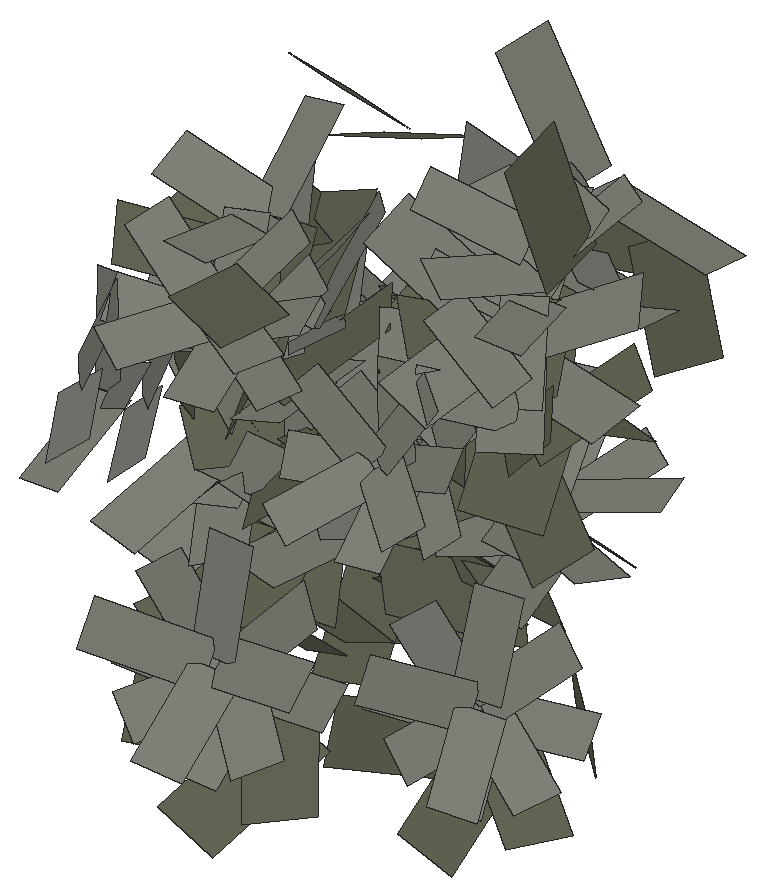
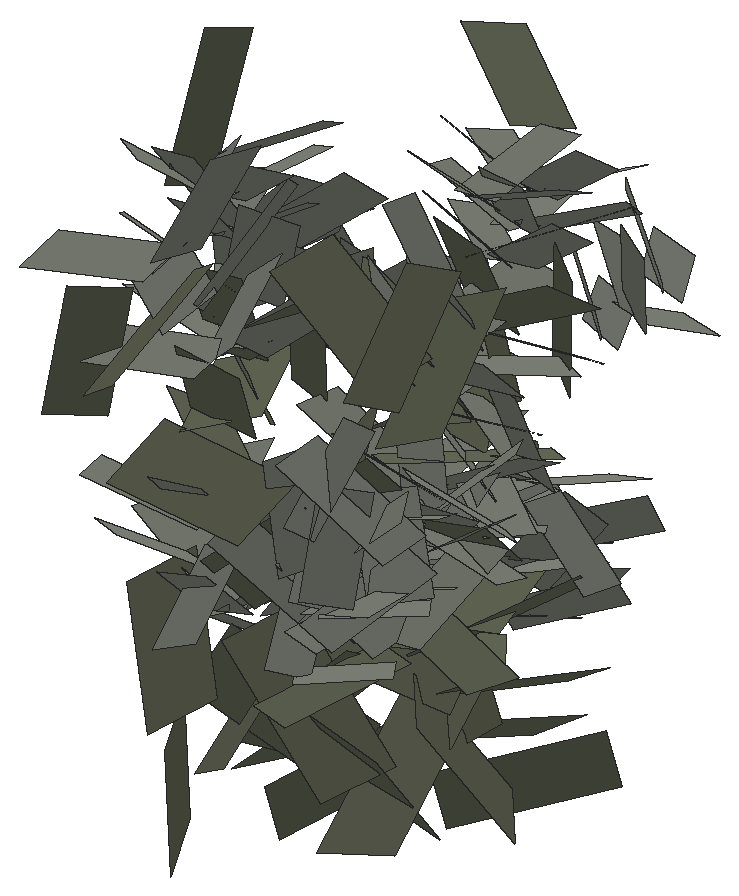
# SketchUp Ruby script. Lengths in inches.
U = 1.inch
M = Sketchup.active_model
def pt(a) = Geom::Point3d.new(a.map { |v| v * U })
def face(e, loops, mat)
  f = e.add_face(loops[0].map { |a| pt(a) })
  loops[1..].each { |l| e.add_face(l.map { |a| pt(a) }).erase! }
  f.material = f.back_material = mat if mat
  f
end
# faces: each face lists its corners as indices into pts; further lists are holes
def faces(e, pts, list, mat = nil) = list.each { |f| face(e, (f[0].is_a?(Array) ? f : [f]).map { |l| l.map { |i| pts[i] } }, mat) }
# xy, xz, yz: faces in a plane at the given z, y or x. An outline is a flat list of corners, or four numbers for a rectangle; further outlines are holes
def ring(l) = l.size == 4 ? [[l[0], l[1]], [l[2], l[1]], [l[2], l[3]], [l[0], l[3]]] : l.each_slice(2).to_a
def flat(e, list, mat, &to3) = list.each { |f| face(e, (f[0].is_a?(Array) ? f : [f]).map { |l| ring(l).map { |u, v| to3.(u, v) } }, mat) }
def xy(e, z, list, mat = nil) = flat(e, list, mat) { |x, y| [x, y, z] }
def xz(e, y, list, mat = nil) = flat(e, list, mat) { |x, z| [x, y, z] }
def yz(e, x, list, mat = nil) = flat(e, list, mat) { |y, z| [x, y, z] }
def lines(e, pts, list) = list.each { |a, b| e.add_line(pt(pts[a]), pt(pts[b])) }
# prism: a flat outline (further loops are holes) pulled along v
def prism(e, loops, v, mat = nil)
  f = face(e, loops, mat); d = Geom::Vector3d.new(v.map { |x| x * U })
  f.pushpull(f.normal.samedirection?(d) ? d.length : -d.length)
end
def box(e, o, s, mat = nil) = prism(e, [[o, [o[0] + s[0], o[1], o[2]], [o[0] + s[0], o[1] + s[1], o[2]], [o[0], o[1] + s[1], o[2]]]], [0, 0, s[2]], mat)
def at(x, y, z, deg = 0) = Geom::Transformation.translation(pt([x, y, z])) * Geom::Transformation.rotation(ORIGIN, Z_AXIS, deg.degrees)
def axes(o, x, y, z) = Geom::Transformation.new([*x, 0, *y, 0, *z, 0, *pt(o).to_a, 1])
def part(name) = M.definitions.add(name)
# library, detail: a bought-in or finely detailed component or shape, given as its bounding box
def library(name, o, s) = part(name).tap { |d| box(d.entities, o, s) }
def detail(e, o, s) = box(e.add_group.entities, o, s)
def put(e, d, t, mat = nil) = e.add_instance(d, t).tap { |i| i.material = mat if mat }
def group(e, t, mat = nil) = e.add_group.tap { |g| g.transformation = t; g.material = mat if mat }.entities
root = M.entities
M.materials.add("viburnumblaasdfas0df1w06d").color = [98, 102, 84]
M.materials.add("viburnumbladsadfasdfad0w122").color = [125, 129, 119]
c1 = part("Component\#315")
p = [[0.25,0,0],[2.05,0.01,0.35],[1.81,4.2,1.66],[0,4.19,1.3125]]
faces(c1.entities,p,[[0,1,2,3]],"viburnumbladsadfasdfad0w122")
c2 = part("viburnumblad2")
put(c2.entities,c1,axes([-19.23,-4.49,-32.18],[83.35428,0,0],[0,79.38502,0],[0,0,83.35428]))
c3 = part("Component\#314")
p = [[0.14,0,0],[2.58,0.05,0.25],[2.44,5.11,2.64],[0,5.05,2.39]]
faces(c3.entities,p,[[0,1,2,3]],"viburnumblaasdfas0df1w06d")
c4 = part("viburnumblad1\#2")
put(c4.entities,c3,axes([-37.25,6.23,19.31],[75.98784,0,0],[0,65.50676,0],[0,0,75.98784]))
put(root,c2,axes([1226.33,274.85,14.94],[0.00016,-0.01206,-0.00411],[0.01207,-0.0013,0.00429],[-0.00443,-0.00391,0.01129]))
put(root,c2,axes([1229.25,283.21,16.14],[-0.01389,0,-0.00185],[-0.00005,-0.01523,0.00032],[-0.00201,0.00032,0.0151]))
put(root,c4,axes([1228.82,284.94,25.53],[-0.01366,0.00026,0.00163],[0.00037,-0.01516,0.00432],[0.00177,0.00434,0.01188]))
put(root,c2,axes([1227.91,269.2,22.33],[0.01118,-0.00278,0.00257],[-0.00082,0.00655,0.0102],[-0.00357,-0.00931,0.00467]))
put(root,c2,axes([1226.33,278.8,18.92],[0.00883,-0.00666,-0.00546],[0.00861,0.00836,0.00373],[0.00207,-0.0066,0.01002]))
put(root,c2,axes([1229.81,277.7,17.24],[0.00207,0.01081,-0.00198],[-0.01024,0.00263,0.00364],[0.00398,0.00114,0.01039]))
put(root,c4,axes([1230.33,279.36,10.75],[-0.01218,0.00376,0.00725],[-0.00872,-0.0119,-0.00846],[0.0032,-0.00977,0.01045]))
put(root,c4,axes([1230.91,277.52,4.82],[-0.00011,0.00616,0.01357],[-0.0165,-0.00475,0.00202],[0.00445,-0.01294,0.00591]))
put(root,c4,axes([1227.07,278.17,5.83],[0.01021,-0.01095,0.0021],[0.01009,0.01114,0.00903],[-0.00698,-0.00405,0.01279]))
put(root,c4,axes([1225.9,281.68,13.5],[-0.00229,-0.01326,-0.00295],[0.0155,-0.0021,-0.00237],[0.00206,-0.00324,0.01267]))
put(root,c2,axes([1230,275.96,15.39],[-0.0137,0.00216,0.00156],[-0.00229,-0.00943,-0.00711],[-0.00005,-0.00804,0.01068]))
put(root,c2,axes([1226.58,279.63,17.48],[0.00038,-0.01114,-0.00561],[0.01301,0.00109,-0.00087],[0.0016,-0.0057,0.01058]))
put(root,c2,axes([1230.72,284.14,17.18],[-0.00604,0.00926,-0.00001],[-0.00892,-0.00582,-0.00295],[-0.00247,-0.0016,0.01066]))
put(root,c2,axes([1231.21,274.45,23.76],[-0.00263,0.0123,0.00535],[-0.01296,-0.00091,-0.00426],[-0.00348,-0.00589,0.01184]))
put(root,c2,axes([1229.125,277.97,15.94],[0.00864,0.00566,-0.00294],[-0.00615,0.01026,0.00169],[0.00342,0.0003,0.01064]))
put(root,c2,axes([1230.12,273.79,17.89],[-0.01312,0.00207,0.00149],[-0.00255,-0.01047,-0.0079],[-0.00005,-0.00804,0.01068]))
put(root,c2,axes([1227.85,278.78,18.53],[-0.00829,-0.0091,-0.00248],[0.00914,-0.00728,-0.00415],[0.002,-0.00468,0.01099]))
put(root,c2,axes([1230.34,285.84,17.18],[-0.01091,0.00229,-0.00461],[-0.00339,-0.01305,0.00154],[-0.00434,0.00249,0.01152]))
put(root,c2,axes([1229.875,268.62,22.7],[-0.01118,0.00278,-0.00257],[-0.00011,-0.00839,-0.00838],[-0.00365,-0.00753,0.00688]))
put(root,c2,axes([1230.76,277.88,18.45],[-0.00607,0.00939,0.00026],[-0.0086,-0.00567,0.00435],[0.00378,0.00216,0.0103]))
put(root,c2,axes([1230.97,283.08,17.18],[0.00229,0.01091,-0.00461],[-0.01305,0.00339,0.00154],[0.00249,0.00434,0.01152]))
put(root,c2,axes([1227.89,274.44,18.43],[0.01312,-0.00207,-0.00149],[0.00246,0.00822,0.01025],[-0.00067,-0.01033,0.00845]))
put(root,c4,axes([1229.13,282.68,22.59],[-0.01489,-0.00148,0.00524],[0.00198,-0.01828,0.00047],[0.00517,0.00094,0.01496]))
put(root,c2,axes([1227.68,268.5625,23.79],[0.00814,-0.00715,-0.0046],[0.00716,0.00216,0.00888],[-0.00455,-0.00881,0.00477]))
put(root,c2,axes([1229.48,278.42,18.7],[0.009,0.00589,-0.00306],[-0.00569,0.0095,0.00156],[0.00342,0.0003,0.01064]))
put(root,c4,axes([1231.67,274.02,22.86],[0.0051,0.011,0.00655],[-0.01483,0.00551,0.0023],[-0.00067,-0.00681,0.01196]))
put(root,c4,axes([1232.05,277.62,10.8],[-0.00702,0.01204,0.00725],[-0.01547,-0.00958,0.00093],[0.00442,-0.0058,0.01392]))
put(root,c2,axes([1228.73,284.16,17.9],[-0.01077,-0.01069,-0.00135],[0.00977,-0.00996,0.00094],[-0.00168,-0.00022,0.01514]))
put(root,c4,axes([1229.32,272.61,20.55],[0.01089,-0.00679,0.00142],[0.00218,0.00667,0.0129],[-0.00665,-0.00902,0.00468]))
put(root,c2,axes([1231.39,284.74,14.59],[-0.0063,0.00967,-0.00001],[-0.00803,-0.00524,-0.00265],[-0.00247,-0.0016,0.01066]))
put(root,c2,axes([1229.08,268.06,23.91],[-0.00766,-0.00322,-0.00823],[0.00764,-0.00813,-0.00386],[-0.0046,-0.00755,0.00633]))
put(root,c2,axes([1231.57,276.66,14.33],[0.00051,0.01437,0.00412],[-0.01266,-0.00025,0.00242],[0.00266,-0.00396,0.0135]))
put(root,c2,axes([1231.73,283.59,18.58],[-0.007,0.00987,-0.00339],[-0.01018,-0.00558,0.00479],[0.00226,0.00542,0.01111]))
put(root,c4,axes([1229.17,280.28,6.07],[0.01682,-0.00022,0.00237],[-0.00091,0.01794,0.00812],[-0.00224,-0.00704,0.0153]))
put(root,c2,axes([1231.18,275.52,22.14],[0.00694,0.00883,0.00779],[-0.01027,0.00714,0.00105],[-0.0037,-0.00696,0.01117]))
put(root,c2,axes([1232.01,275.5,17.65],[0.00048,0.01376,0.00394],[-0.01406,-0.00028,0.00269],[0.00266,-0.00396,0.0135]))
put(root,c2,axes([1229.83,286.6,18.58],[-0.00987,-0.007,-0.00339],[0.00558,-0.01018,0.00479],[-0.00542,0.00226,0.01111]))
put(root,c2,axes([1231.8,272.82,28.14],[0.00044,0.0126,0.00361],[-0.0113,0.00031,0.00032],[0.00024,-0.00347,0.01207]))
put(root,c2,axes([1232.23,276.08,20.97],[-0.00274,0.01284,0.00559],[-0.01166,-0.00082,-0.00384],[-0.00348,-0.00589,0.01184]))
put(root,c4,axes([1230.46,284.3,6.45],[-0.01776,-0.00139,0.00308],[0.00179,-0.02087,0.00087],[0.003,0.001,0.0178]))
put(root,c4,axes([1228.36,278.68,13.14],[0.01107,-0.00525,0.00049],[0.00612,0.01279,-0.0012],[0,0.00115,0.01221]))
put(root,c4,axes([1232.75,273.61,25.15],[-0.0066,0.01089,0.00527],[-0.0139,-0.00777,-0.00135],[0.00164,-0.00514,0.01268]))
put(root,c2,axes([1228.74,269.65,23.34],[0.00034,-0.00733,-0.00907],[0.00978,-0.00348,0.00299],[-0.00497,-0.00808,0.00546]))
put(root,c2,axes([1230.03,275.71,23.9],[0.01244,0.00019,0.00567],[-0.00322,0.01148,0.00668],[-0.00467,-0.00741,0.01049]))
put(root,c2,axes([1231.07,278.27,16.84],[-0.01065,0.00247,0.00234],[-0.00174,-0.01065,0.00331],[0.00294,0.00276,0.01043]))
put(root,c2,axes([1228.8,270.61,22.42],[0.0085,-0.00746,-0.0048],[0.00645,0.00195,0.00799],[-0.00455,-0.00881,0.00477]))
put(root,c2,axes([1232.09,271.56,10.17],[-0.00011,0.00779,0.00854],[-0.01208,-0.00262,0.00224],[0.00345,-0.0089,0.00816]))
put(root,c2,axes([1227.92,284.33,19.89],[0,-0.01516,-0.00154],[0.01507,-0.00022,0.00221],[-0.00223,-0.00152,0.015]))
put(root,c2,axes([1228.24,284.51,16.125],[0,-0.01583,-0.00161],[0.01357,-0.0002,0.00199],[-0.00223,-0.00152,0.015]))
put(root,c2,axes([1231.55,285.12,16.15],[-0.01032,0.0026,-0.00299],[-0.00231,-0.01123,-0.0018],[-0.0033,-0.001,0.0105]))
put(root,c2,axes([1229.9,275.68,17.3125],[-0.01106,-0.0052,-0.00541],[0.00776,-0.00965,-0.0066],[-0.00127,-0.0082,0.01048]))
put(root,c2,axes([1229.21,278.8125,17.22],[0.01065,-0.00247,-0.00234],[0.00251,0.01145,-0.00069],[0.00243,0.00013,0.01091]))
put(root,c2,axes([1232.61,275.64,22.875],[-0.01065,0.00857,-0.00023],[-0.00787,-0.00997,-0.00669],[-0.00415,-0.00484,0.01209]))
put(root,c4,axes([1233.78,278.32,15.75],[0.00121,0.01104,0.01007],[-0.01675,0.00403,-0.00241],[-0.00386,-0.00953,0.01091]))
put(root,c2,axes([1231.18,276.36,16.01],[0.01044,0.00958,0.00206],[-0.00879,0.00856,0.00474],[0.00211,-0.00514,0.0132]))
put(root,c2,axes([1232.86,276.46,15.95],[-0.00976,0.00988,0.00351],[-0.01076,-0.01049,-0.00039],[0.00219,-0.00277,0.01388]))
put(root,c2,axes([1229.97,270.15,22.62],[-0.00655,-0.0022,-0.00816],[0.00764,-0.00813,-0.00386],[-0.0054,-0.00785,0.00541]))
put(root,c4,axes([1230.25,278.77,13.42],[-0.01365,-0.00518,-0.0014],[0.0059,-0.01311,-0.00908],[0.00168,-0.00777,0.01232]))
put(root,c2,axes([1228.44,275.99,17.59],[0.00749,-0.00812,-0.00752],[0.01093,0.00403,0.00654],[-0.00171,-0.00982,0.0089]))
put(root,c2,axes([1232.49,269.22,12.02],[0.00026,0.00745,0.01011],[-0.01208,-0.00262,0.00224],[0.00344,-0.00977,0.00711]))
put(root,c2,axes([1231.48,270.58,11.4],[0.00896,0.00627,0.00619],[-0.00837,0.00305,0.00903],[0.00298,-0.01046,0.00629]))
put(root,c4,axes([1232.73,285.58,12.23],[-0.011,0.00511,-0.00003],[-0.00581,-0.01252,-0.00271],[-0.00101,-0.0021,0.0119]))
put(root,c2,axes([1232.85,269.78,25.04],[-0.00261,0.00974,0.006],[-0.01123,-0.00353,0.00072],[0.00254,-0.00551,0.00899]))
put(root,c2,axes([1232.17,270.71,24.1],[0.00601,0.00853,0.00433],[-0.01051,0.00446,0.00545],[0.00235,-0.00645,0.00846]))
put(root,c2,axes([1232.1,269.15,26.35],[0.00626,0.00889,0.00451],[-0.00973,0.00413,0.00504],[0.00235,-0.00645,0.00846]))
put(root,c4,axes([1229.4375,278.43,8.47],[-0.00936,-0.00715,0.0061],[0.00985,-0.01174,0.00135],[0.00403,0.00472,0.01172]))
put(root,c4,axes([1234.13,277.57,18.41],[-0.01024,0.01003,0.00441],[-0.01249,-0.0094,-0.00763],[-0.00202,-0.00765,0.01274]))
put(root,c4,axes([1228.52,283.75,25.59],[-0.00484,-0.01365,0.00231],[0.016,-0.00575,-0.00049],[0.00117,0.00203,0.01447]))
put(root,c2,axes([1230.64,278.92,15.56],[-0.00842,-0.00565,0.00174],[0.00635,-0.00914,0.00106],[0.00096,0.00194,0.01097]))
put(root,c4,axes([1231.02,276.02,20.64],[0.01421,-0.00084,0.00442],[-0.0012,0.01582,0.00687],[-0.00438,-0.00595,0.01294]))
put(root,c2,axes([1232.34,284.63,19.83],[-0.01229,0.00259,0.00001],[-0.00225,-0.0107,0.00618],[0.00128,0.00604,0.01094]))
put(root,c2,axes([1229.17,277.08,16.37],[-0.00242,-0.00904,-0.00878],[0.01402,-0.00344,-0.00033],[-0.00196,-0.00893,0.00974]))
put(root,c2,axes([1231.15,277.07,21.14],[0.01184,0.00091,0.00415],[-0.00322,0.01148,0.00668],[-0.0033,-0.00735,0.01104]))
put(root,c2,axes([1229.42,274.91,18.94],[-0.00252,-0.00942,-0.00914],[0.01298,-0.00318,-0.00031],[-0.00196,-0.00893,0.00974]))
put(root,c2,axes([1229.51,279.32,15.7],[0.00633,-0.0098,-0.00027],[0.00833,0.00542,-0.00155],[0.00159,0.00072,0.01104]))
put(root,c2,axes([1231.17,285.39,17.62],[-0.00856,-0.00558,-0.00422],[0.00556,-0.00947,0.00126],[-0.00425,-0.00115,0.01014]))
put(root,c4,axes([1228.69,279.24,10.95],[0.00308,-0.0114,0.00333],[0.01375,0.00318,-0.00182],[0.00071,0.00361,0.0117]))
put(root,c2,axes([1233.23,270.8,11.1875],[-0.00859,0.00427,0.00811],[-0.00794,-0.00683,-0.00482],[0.00302,-0.00917,0.00803]))
put(root,c4,axes([1232.6,276.16,6.97],[-0.01186,-0.00066,0.00699],[-0.00532,-0.01121,-0.01007],[0.00532,-0.0098,0.0081]))
put(root,c2,axes([1232.3,275.37,24.74],[-0.01244,-0.00019,-0.00567],[0.00199,-0.01294,-0.00394],[-0.00531,-0.00441,0.0118]))
put(root,c2,axes([1230.67,277.8125,14.84],[0.01298,0.00037,-0.00224],[0.00059,0.01317,0.00559],[0.0024,-0.0056,0.01296]))
put(root,c2,axes([1230.21,279.59,16.85],[-0.00207,-0.01081,0.00198],[0.01001,-0.00209,-0.00093],[0.00139,0.00174,0.01096]))
put(root,c2,axes([1231.24,279.17,18.16],[-0.009,-0.00589,0.00306],[0.00635,-0.00914,0.00106],[0.00195,0.00259,0.0107]))
put(root,c4,axes([1229.22,285.53,9.72],[-0.00613,-0.01546,0.00166],[0.01796,-0.00686,0.00247],[-0.00138,0.00232,0.01649]))
put(root,c2,axes([1230.99,273.87,28.45],[0.01156,-0.00022,-0.00012],[0.00026,0.01157,0.0049],[0.00003,-0.0049,0.01157]))
put(root,c2,axes([1229.96,279.71,18.4],[0.00607,-0.00939,-0.00026],[0.00926,0.00603,-0.00173],[0.00159,0.00072,0.01104]))
put(root,c2,axes([1231.74,286.05,14.97],[-0.00821,-0.00536,-0.00406],[0.00601,-0.01023,0.00136],[-0.00425,-0.00115,0.01014]))
put(root,c4,axes([1231.34,273.01,22.41],[0.01287,-0.00107,0.00071],[0.00034,0.01171,0.00907],[-0.00141,-0.0079,0.00892]))
put(root,c2,axes([1233.59,269.3,26.27],[-0.00995,0.00489,0.00397],[-0.00607,-0.00954,-0.00338],[0.0019,-0.00477,0.00949]))
put(root,c2,axes([1233,277.79,14.51],[-0.01371,0.0002,0.00098],[-0.0004,-0.01527,-0.00242],[0.00098,-0.00226,0.01411]))
put(root,c2,axes([1231.02,276.93,18.14],[0.01428,-0.00021,-0.00102],[0.00059,0.01317,0.00559],[0.00086,-0.00561,0.01315]))
put(root,c2,axes([1233.05,273.75,28.49],[-0.01199,0.00073,-0.00108],[-0.00063,-0.01339,-0.00213],[-0.00123,-0.0019,0.01236]))
put(root,c4,axes([1230.57,274.58,20.49],[0.00428,-0.01029,-0.00658],[0.01194,-0.00078,0.00879],[-0.00649,-0.00737,0.00685]))
put(root,c2,axes([1231.79,270.43,25.51],[0.01146,0.00283,0.00038],[-0.00257,0.0094,0.00741],[0.00146,-0.00704,0.00821]))
put(root,c2,axes([1230.79,277.23,22.93],[0.01065,-0.00857,0.00023],[0.00633,0.00812,0.0092],[-0.00584,-0.00699,0.01019]))
put(root,c2,axes([1233.15,272.25,10.67],[-0.01296,-0.00148,0.00142],[-0.00002,-0.00776,-0.00823],[0.00196,-0.00903,0.00851]))
put(root,c4,axes([1233.6,280.8,13.54],[0.01304,-0.00033,0.00964],[-0.00605,0.01553,0.00873],[-0.00811,-0.00915,0.01066]))
put(root,c2,axes([1233.52,276.48,17.84],[-0.01428,0.00021,0.00102],[-0.00037,-0.01414,-0.00224],[0.00098,-0.00226,0.01411]))
put(root,c2,axes([1231.62,269.89,13.17],[0.01241,0.00141,-0.00136],[0.00049,0.00618,0.01093],[0.0019,-0.01085,0.00605]))
put(root,c2,axes([1233.24,277.13,21.93],[-0.01194,-0.00018,-0.00545],[0.00215,-0.01397,-0.00426],[-0.00531,-0.00441,0.0118]))
put(root,c2,axes([1232.27,284.98,17.97],[-0.01038,-0.0062,0.0034],[0.00714,-0.00931,0.00482],[0.00014,0.00586,0.01111]))
put(root,c2,axes([1231.125,276.625,24.875],[0.00263,-0.0123,-0.00535],[0.01173,-0.00054,0.007],[-0.00651,-0.00594,0.01045]))
put(root,c2,axes([1233.79,269.91,12.62],[-0.01241,-0.00141,0.00136],[-0.00002,-0.00862,-0.00914],[0.00196,-0.00903,0.00851]))
put(root,c4,axes([1235.05,281.62,7.9375],[0.0025,0.01316,0.00583],[-0.01545,-0.00015,0.00696],[0.00546,-0.00635,0.01198]))
put(root,c2,axes([1231.41,284.98,16.52],[-0.00213,-0.01089,0.00325],[0.01232,-0.002,0.0014],[-0.00076,0.00372,0.01198]))
put(root,c4,axes([1235.48,282.8,14.21],[0.00442,0.01183,0.01203],[-0.01827,-0.00182,0.0085],[0.00605,-0.01272,0.01028]))
put(root,c2,axes([1232.42,277.02,23.55],[-0.00694,-0.00883,-0.00779],[0.00996,-0.00923,0.0016],[-0.00629,-0.00487,0.01112]))
put(root,c4,axes([1232.12,283.44,15.36],[-0.01205,-0.00086,0.01408],[0.00278,-0.02131,0.00108],[0.0139,0.00242,0.01204]))
put(root,c2,axes([1233.84,270.82,25.53],[-0.01146,-0.00283,-0.00038],[0.00275,-0.01049,-0.00491],[0.00082,-0.00467,0.00968]))
put(root,c2,axes([1231.97,271.95,24.9],[0.01038,-0.0051,-0.00415],[0.00572,0.00729,0.00502],[0.00038,-0.00694,0.0084]))
put(root,c2,axes([1231.25,278.29,16.61],[0.00976,-0.00988,-0.00351],[0.01058,0.00912,0.00376],[-0.00035,-0.00511,0.01338]))
put(root,c4,axes([1230.84,282.71,8.77],[-0.00166,-0.01224,0.00834],[0.01717,-0.00122,0.00163],[-0.00056,0.00844,0.01227]))
put(root,c4,axes([1232.74,275.85,19.44],[-0.00918,-0.00626,-0.00848],[0.01129,-0.01094,-0.00412],[-0.00395,-0.00772,0.00939]))
put(root,c2,axes([1232.03,270.43,27.11],[0.00995,-0.00489,-0.00397],[0.00635,0.0081,0.00558],[0.00038,-0.00694,0.0084]))
put(root,c2,axes([1231.75,271.54,12.66],[0.00859,-0.00427,-0.00811],[0.00913,0.005,0.00703],[0.00084,-0.0107,0.00653]))
put(root,c4,axes([1232.7,275.16,9.32],[-0.01126,-0.00753,-0.00255],[0.00827,-0.00884,-0.01044],[0.00351,-0.00867,0.01012]))
put(root,c4,axes([1231.57,275.07,21.39],[0.0077,-0.00971,-0.00377],[0.01191,0.00736,0.00523],[-0.00177,-0.00557,0.01033]))
put(root,c2,axes([1233.06,278,16.41],[-0.01044,-0.00958,-0.00206],[0.0098,-0.01029,-0.00181],[-0.00027,-0.00273,0.01406]))
put(root,c4,axes([1235.23,281.32,4.53],[-0.00036,0.00539,0.01277],[-0.01275,-0.00915,0.0035],[0.00843,-0.01005,0.00448]))
put(root,c2,axes([1233.14,271.65,12.4],[-0.00896,-0.00627,-0.00619],[0.0092,-0.00573,-0.00751],[0.00088,-0.00942,0.00827]))
put(root,c2,axes([1232.43,271.52,26.07],[0.00261,-0.00974,-0.006],[0.01057,0.00192,0.00135],[-0.00026,-0.0062,0.0089]))
put(root,c2,axes([1232.14,272.89,11.74],[-0.00025,-0.00716,-0.0097],[0.01356,0.0002,-0.00049],[0.00042,-0.01011,0.00745]))
put(root,c2,axes([1233.23,272.08,24.93],[-0.00572,-0.00761,-0.00506],[0.01001,-0.00557,-0.00285],[-0.00075,-0.00619,0.00889]))
put(root,c4,axes([1235.39,285.26,8.43],[-0.01278,0.00636,0.00656],[-0.00548,-0.01653,0.00535],[0.00782,0.00178,0.01351]))
put(root,c2,axes([1233.51,270.57,27.03],[-0.00626,-0.00889,-0.00451],[0.01001,-0.00557,-0.00285],[-0.00007,-0.00526,0.00943]))
put(root,c2,axes([1232.53,277.91,18.32],[-0.00048,-0.01376,-0.00394],[0.01429,-0.00069,0.00066],[-0.00082,-0.00391,0.01375]))
put(root,c2,axes([1232.92,270.58,13.76],[-0.00026,-0.00745,-0.01011],[0.01255,0.00018,-0.00046],[0.00042,-0.01011,0.00745]))
put(root,c4,axes([1232.83,276.46,19.46],[-0.00628,-0.01206,-0.00336],[0.01448,-0.00668,-0.00311],[0.00091,-0.00388,0.01211]))
put(root,c4,axes([1236.89,281.75,9.93],[-0.00888,0.00849,0.00791],[-0.01054,-0.01309,0.0022],[0.00721,-0.00377,0.01214]))
put(root,c2,axes([1237.17,280.76,13.2],[-0.00337,0.01279,0.00428],[-0.0107,-0.00403,0.00361],[0.00507,-0.00269,0.01202]))
put(root,c4,axes([1233.54,269.74,28.38],[-0.00662,-0.01127,-0.00498],[0.01432,-0.00702,-0.0031],[-0.00011,-0.00548,0.01154]))
put(root,c2,axes([1236.76,286.43,14.33],[-0.01437,0.00051,0.00412],[0.00025,-0.01266,0.00242],[0.00396,0.00266,0.0135]))
put(root,c2,axes([1237.11,280.38,14.79],[0.0065,0.01157,0.00112],[-0.00968,0.00489,0.00566],[0.0049,-0.00389,0.01176]))
put(root,c2,axes([1238.04,272.59,20.04],[-0.00143,0.00635,0.00868],[-0.0108,-0.00196,-0.00037],[0.00136,-0.00839,0.00553]))
put(root,c2,axes([1237.23,271.65,20.95],[0.00668,0.00514,0.00687],[-0.00864,0.00277,0.00603],[0.00109,-0.00897,0.00475]))
put(root,c2,axes([1238.28,279.87,16.18],[-0.00323,0.01225,0.0041],[-0.01189,-0.00447,0.00401],[0.00507,-0.00269,0.01202]))
put(root,c2,axes([1238.1,278.0625,21.99],[0.00298,0.01174,0.00601],[-0.01309,-0.0001,0.00669],[0.00586,-0.00729,0.01134]))
put(root,c2,axes([1237.56,273.82,19.61],[0.00642,0.00493,0.0066],[-0.00933,0.00299,0.00651],[0.00109,-0.00897,0.00475]))
put(root,c4,axes([1237.97,281.84,16.59],[-0.01126,0.00378,0.01091],[-0.00977,-0.0152,-0.00482],[0.00789,-0.0086,0.01113]))
put(root,c2,axes([1236.1,281.51,13.8125],[0.01096,0.00423,-0.00348],[-0.00277,0.01177,0.00559],[0.00527,-0.00421,0.01149]))
put(root,c2,axes([1238.16,282.06,25.57],[-0.00842,0.01125,0.00685],[-0.00786,-0.01092,0.00827],[0.01063,0.001,0.01143]))
put(root,c2,axes([1238.54,280.97,14.55],[-0.01106,0.00576,0.00468],[-0.00631,-0.01247,0.00042],[0.00435,-0.00178,0.01246]))
put(root,c4,axes([1233.21,284.99,18.66],[-0.00321,-0.01557,0.00645],[0.01613,-0.00714,-0.00921],[0.00952,0.00374,0.01377]))
put(root,c2,axes([1238.62,271.63,20.89],[-0.00871,0.00384,0.00541],[-0.00663,-0.00614,-0.00616],[0.00084,-0.00787,0.00624]))
put(root,c4,axes([1239.03,278.47,20.96],[0.00193,0.01121,0.0059],[-0.01433,0.00039,0.00396],[0.00283,-0.0062,0.01085]))
put(root,c2,axes([1238.38,281.88,27.91],[0.00042,0.01563,0.00009],[-0.01107,0.00024,0.01104],[0.01103,-0.00036,0.01108]))
put(root,c2,axes([1237.49,283.14,23.89],[-0.01223,0.0001,0.00757],[0.00075,-0.01555,0.00142],[0.00819,0.0016,0.01322]))
put(root,c2,axes([1238.66,276.43,9.12],[-0.00143,0.00682,0.00818],[-0.0095,-0.00594,0.0033],[0.00662,-0.0068,0.00682]))
put(root,c2,axes([1238.98,276.12,24.79],[0.00385,0.0119,0.00772],[-0.01309,-0.0001,0.00669],[0.00547,-0.00863,0.01057]))
put(root,c4,axes([1237.36,280.63,6.27],[-0.00935,-0.00415,0.00773],[-0.00246,-0.01147,-0.00913],[0.00851,-0.00702,0.00652]))
put(root,c4,axes([1235.8,286.92,10.8],[-0.01204,-0.00702,0.00725],[0.00958,-0.01547,0.00093],[0.0058,0.00442,0.01392]))
put(root,c4,axes([1237.62,280.03,19.06],[0.01317,0.00353,0.00249],[-0.00497,0.01356,0.00706],[-0.00054,-0.00655,0.0122]))
put(root,c2,axes([1237.04,280.84,16.78],[0.01242,0.00411,-0.00252],[-0.00277,0.01177,0.00559],[0.00395,-0.00468,0.01183]))
put(root,c2,axes([1237.125,273.09,20.71],[0.01089,0.00092,0.00104],[-0.00149,0.00552,0.00975],[0.0002,-0.00927,0.00435]))
put(root,c2,axes([1239.64,277.43,23.07],[-0.00693,0.00909,0.00924],[-0.01085,-0.00802,-0.00026],[0.00532,-0.00757,0.01142]))
put(root,c2,axes([1237.73,277.54,23.86],[0.01238,0.00774,0.00167],[-0.00648,0.00805,0.01066],[0.00465,-0.00962,0.01009]))
put(root,c4,axes([1237.13,276.52,19.03],[0.0117,-0.0027,-0.00014],[0.00141,0.00653,0.01192],[-0.00257,-0.00994,0.00471]))
put(root,c4,axes([1235.9,285.77,4.82],[-0.00616,-0.00011,0.01357],[0.00475,-0.0165,0.00202],[0.01294,0.00445,0.00591]))
put(root,c2,axes([1238.1,282.18,13.25],[-0.01192,-0.00395,0.00242],[0.00393,-0.01356,-0.00276],[0.00316,-0.0017,0.01283]))
put(root,c2,axes([1238.57,275.38,10.28],[0.00667,0.00821,0.00496],[-0.00717,0.00016,0.00937],[0.00645,-0.00831,0.00509]))
put(root,c2,axes([1239.48,278.84,21.96],[-0.01426,0.00099,0.00559],[-0.00302,-0.01157,-0.00566],[0.00428,-0.00706,0.01216]))
put(root,c2,axes([1240.11,277.45,25.77],[-0.00295,0.01122,0.00376],[-0.00992,-0.00313,0.00154],[0.00265,-0.00298,0.01098]))
put(root,c2,axes([1239.06,273.18,20.8125],[-0.01089,-0.00092,-0.00104],[0.00144,-0.00742,-0.00803],[-0.00015,-0.00772,0.00646]))
put(root,c2,axes([1239.93,274.49,10.69],[-0.00083,0.00664,0.00958],[-0.0095,-0.00594,0.0033],[0.00675,-0.00756,0.00582]))
put(root,c4,axes([1239.4,286.53,22.86],[-0.011,0.0051,0.00655],[-0.00551,-0.01483,0.0023],[0.00681,-0.00067,0.01196]))
put(root,c2,axes([1236.67,282.1,15.4],[0.01106,-0.00576,-0.00468],[0.00696,0.01121,0.00265],[0.00276,-0.0046,0.01219]))
put(root,c4,axes([1240.36,278.43,22.94],[-0.0084,0.0076,0.00599],[-0.00998,-0.01102,-0.00002],[0.00443,-0.00403,0.01133]))
put(root,c2,axes([1240.64,276.52,28.47],[-0.00283,0.01075,0.0036],[-0.01102,-0.00348,0.00171],[0.00265,-0.00298,0.01098]))
put(root,c2,axes([1240,276.11,9.9],[-0.00784,0.00117,0.00859],[-0.00546,-0.0084,-0.00383],[0.00631,-0.00716,0.00674]))
put(root,c2,axes([1236.64,284.49,24.4375],[-0.00044,-0.01632,-0.00009],[0.01207,-0.00029,-0.00723],[0.00803,-0.00029,0.01342]))
put(root,c2,axes([1239.83,277.0625,27.125],[0.00596,0.00978,0.00229],[-0.00894,0.00456,0.00379],[0.00249,-0.00402,0.01069]))
put(root,c2,axes([1237.29,272.46,22.05],[0.00871,-0.00384,-0.00541],[0.00664,0.00406,0.00749],[-0.00079,-0.00912,0.00457]))
put(root,c2,axes([1237.49,274.61,20.74],[0.00909,-0.00401,-0.00564],[0.00597,0.00365,0.00674],[-0.00079,-0.00912,0.00457]))
put(root,c2,axes([1239.44,277.36,9.49],[-0.01071,-0.0052,0.00268],[0.00135,-0.00683,-0.00788],[0.0054,-0.00736,0.0073]))
put(root,c2,axes([1239.33,281.1875,16.22],[-0.01242,-0.00411,0.00252],[0.00364,-0.01255,-0.00256],[0.00316,-0.0017,0.01283]))
put(root,c2,axes([1238.19,284.27,25.54],[-0.00902,-0.01086,0.00673],[0.00875,-0.01029,-0.00487],[0.0085,0.00104,0.01308]))
put(root,c2,axes([1239.68,282.99,26.92],[-0.01234,0.00028,0.00961],[0.00075,-0.01555,0.00142],[0.00958,0.00158,0.01226]))
put(root,c2,axes([1240.67,276.89,24.8],[-0.01366,0.00095,0.00535],[-0.00336,-0.01286,-0.00628],[0.00428,-0.00706,0.01216]))
put(root,c2,axes([1240.6,275.7,21.93],[0.0032,0.00932,0.00366],[-0.00988,0.00076,0.00635],[0.00496,-0.00497,0.00731]))
put(root,c2,axes([1239.14,278.13,26.1875],[0.01014,0.00329,-0.00138],[-0.00265,0.01026,0.00493],[0.00283,-0.00431,0.01049]))
put(root,c2,axes([1237.83,273.74,21.56],[0.00143,-0.00635,-0.00868],[0.00992,-0.00012,0.00155],[-0.0013,-0.00861,0.00528]))
put(root,c2,axes([1241.13,277.52,27.13],[-0.00997,0.00542,0.0028],[-0.00605,-0.01063,-0.00096],[0.002,-0.00216,0.01131]))
put(root,c4,axes([1238.99,277.48,20.54],[0.01164,0.00293,-0.00079],[-0.00215,0.01041,0.00877],[0.00216,-0.00738,0.00809]))
put(root,c2,axes([1238.67,272.44,22],[-0.00668,-0.00514,-0.00687],[0.00865,-0.00485,-0.0047],[-0.00103,-0.00803,0.00606]))
put(root,c2,axes([1238.68,274.55,20.78],[-0.00601,-0.0039,-0.00689],[0.00865,-0.00485,-0.0047],[-0.00175,-0.00854,0.00529]))
put(root,c4,axes([1238.74,281.6,19.48],[-0.01393,-0.0074,0.00333],[0.00558,-0.01491,-0.00981],[0.00654,-0.00631,0.01332]))
put(root,c4,axes([1237.63,278.63,18.92],[0.00605,-0.00776,-0.00693],[0.01168,0.0029,0.00677],[-0.00267,-0.00844,0.00676]))
put(root,c2,axes([1238.31,282.38,15.01],[-0.0065,-0.01157,-0.00112],[0.01142,-0.00611,-0.00313],[0.00221,-0.00249,0.0129]))
put(root,c4,axes([1238.02,279.78,8.4],[-0.00788,-0.01001,-0.0014],[0.00865,-0.00529,-0.01087],[0.00682,-0.00657,0.00863]))
put(root,c2,axes([1239.1,274.82,11.87],[0.01026,0.00498,-0.00256],[-0.00015,0.00559,0.01026],[0.0056,-0.00897,0.00496]))
put(root,c2,axes([1241.58,275.09,22.68],[-0.00449,0.00779,0.00619],[-0.00867,-0.00648,0.00177],[0.0049,-0.00408,0.00781]))
put(root,c2,axes([1238.38,277.42,25.98],[0.01366,-0.00095,-0.00535],[0.00429,0.01077,0.00904],[0.00334,-0.00996,0.01028]))
put(root,c2,axes([1241.27,274.32,23.96],[0.00334,0.0097,0.00381],[-0.00915,0.00071,0.00588],[0.00496,-0.00497,0.00731]))
put(root,c2,axes([1238.09,282.15,16.82],[0.00323,-0.01225,-0.0041],[0.01276,0.00369,-0.00099],[0.00204,-0.00369,0.01263]))
put(root,c2,axes([1239.97,278.82,24.04],[-0.01238,-0.00774,-0.00167],[0.00772,-0.01057,-0.00819],[0.00296,-0.0074,0.01235]))
put(root,c2,axes([1238.66,276.31,11.45],[0.00784,-0.00117,-0.00859],[0.00729,0.00715,0.00568],[0.00468,-0.00917,0.00553]))
put(root,c2,axes([1238.49,277.62,10.61],[0.00079,-0.00637,-0.0092],[0.01172,0.00425,-0.00193],[0.00425,-0.00877,0.00644]))
put(root,c2,axes([1240.52,275.34,23.26],[0.0092,0.00594,-0.0008],[-0.00419,0.00749,0.00747],[0.00433,-0.00576,0.00715]))
put(root,c2,axes([1240.93,275.49,11.125],[-0.01026,-0.00498,0.00256],[0.0015,-0.00759,-0.00876],[0.0054,-0.00736,0.0073]))
put(root,c4,axes([1238.46,279.36,19.66],[0.00918,-0.00623,-0.00469],[0.00881,0.01006,0.00379],[0.00131,-0.00544,0.00952]))
put(root,c4,axes([1239.02,280.4,17.76],[-0.00713,-0.00827,-0.00706],[0.01264,-0.00623,-0.00545],[-0.00006,-0.00799,0.0088]))
put(root,c2,axes([1240.97,278.64,26],[-0.01081,-0.00296,0.00035],[0.0032,-0.01197,-0.0024],[0.00093,-0.00205,0.01147]))
put(root,c2,axes([1239.8125,276.83,11.06],[-0.00667,-0.00821,-0.00496],[0.00888,-0.00228,-0.00816],[0.00454,-0.00802,0.00718]))
put(root,c2,axes([1238.72,280.1,23.11],[-0.0037,-0.01142,-0.00741],[0.01514,-0.00214,-0.00425],[0.00214,-0.0084,0.01187]))
put(root,c2,axes([1238.48,279.03,24.74],[0.00693,-0.00909,-0.00924],[0.01276,0.00664,0.00304],[0.0023,-0.00946,0.01102]))
put(root,c2,axes([1239.44,278.57,27.66],[0.00997,-0.00542,-0.0028],[0.00614,0.00939,0.00366],[0.00055,-0.00455,0.01075]))
put(root,c4,axes([1240.8125,284.18,20.55],[0.00679,0.01089,0.00142],[-0.00667,0.00218,0.0129],[0.00902,-0.00665,0.00468]))
put(root,c2,axes([1238.83,284.62,27.63],[-0.00042,-0.01563,-0.00009],[0.01341,-0.00032,-0.00803],[0.00803,-0.00029,0.01342]))
put(root,c4,axes([1241.1,277.67,26.83],[0.00008,0.01316,0.00435],[-0.00745,-0.00443,0.01354],[0.01228,-0.00208,0.00607]))
